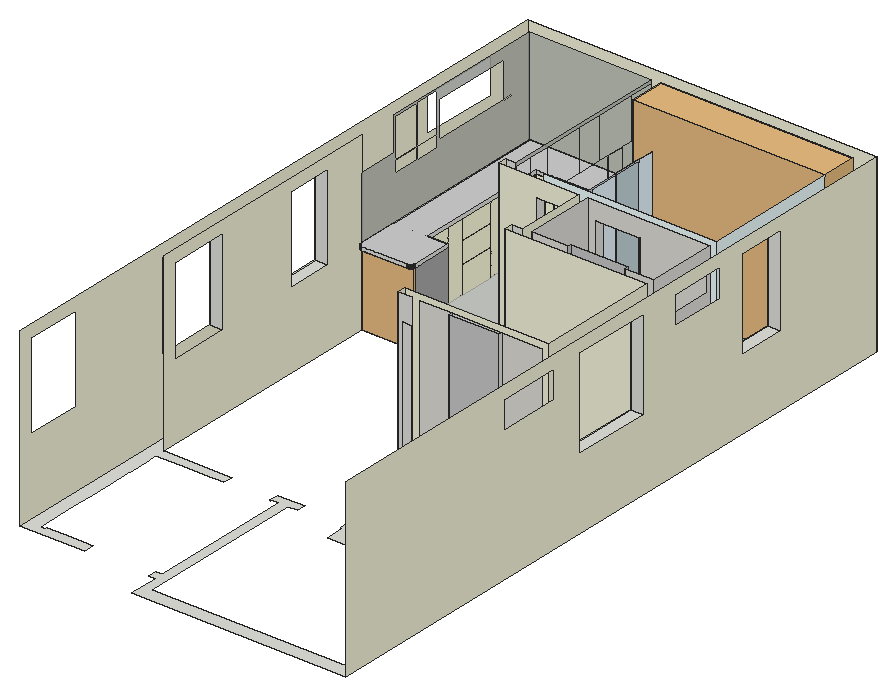
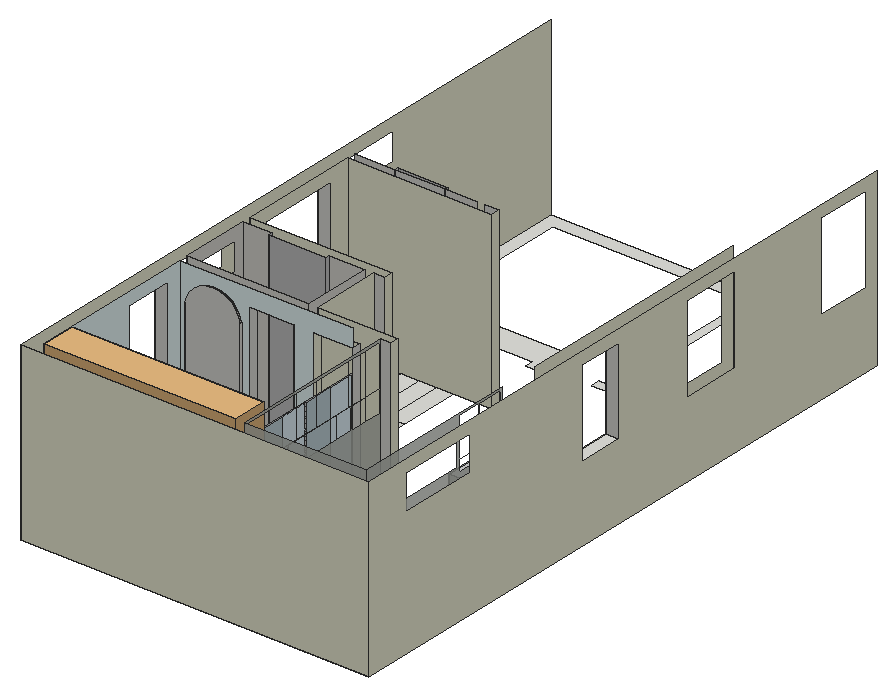
# SketchUp Ruby script. Lengths in inches.
U = 1.inch
M = Sketchup.active_model
def pt(a) = Geom::Point3d.new(a.map { |v| v * U })
def face(e, loops, mat)
  f = e.add_face(loops[0].map { |a| pt(a) })
  loops[1..].each { |l| e.add_face(l.map { |a| pt(a) }).erase! }
  f.material = f.back_material = mat if mat
  f
end
# faces: each face lists its corners as indices into pts; further lists are holes
def faces(e, pts, list, mat = nil) = list.each { |f| face(e, (f[0].is_a?(Array) ? f : [f]).map { |l| l.map { |i| pts[i] } }, mat) }
# xy, xz, yz: faces in a plane at the given z, y or x. An outline is a flat list of corners, or four numbers for a rectangle; further outlines are holes
def ring(l) = l.size == 4 ? [[l[0], l[1]], [l[2], l[1]], [l[2], l[3]], [l[0], l[3]]] : l.each_slice(2).to_a
def flat(e, list, mat, &to3) = list.each { |f| face(e, (f[0].is_a?(Array) ? f : [f]).map { |l| ring(l).map { |u, v| to3.(u, v) } }, mat) }
def xy(e, z, list, mat = nil) = flat(e, list, mat) { |x, y| [x, y, z] }
def xz(e, y, list, mat = nil) = flat(e, list, mat) { |x, z| [x, y, z] }
def yz(e, x, list, mat = nil) = flat(e, list, mat) { |y, z| [x, y, z] }
def lines(e, pts, list) = list.each { |a, b| e.add_line(pt(pts[a]), pt(pts[b])) }
# prism: a flat outline (further loops are holes) pulled along v
def prism(e, loops, v, mat = nil)
  f = face(e, loops, mat); d = Geom::Vector3d.new(v.map { |x| x * U })
  f.pushpull(f.normal.samedirection?(d) ? d.length : -d.length)
end
def box(e, o, s, mat = nil) = prism(e, [[o, [o[0] + s[0], o[1], o[2]], [o[0] + s[0], o[1] + s[1], o[2]], [o[0], o[1] + s[1], o[2]]]], [0, 0, s[2]], mat)
def at(x, y, z, deg = 0) = Geom::Transformation.translation(pt([x, y, z])) * Geom::Transformation.rotation(ORIGIN, Z_AXIS, deg.degrees)
def axes(o, x, y, z) = Geom::Transformation.new([*x, 0, *y, 0, *z, 0, *pt(o).to_a, 1])
def part(name) = M.definitions.add(name)
# library, detail: a bought-in or finely detailed component or shape, given as its bounding box
def library(name, o, s) = part(name).tap { |d| box(d.entities, o, s) }
def detail(e, o, s) = box(e.add_group.entities, o, s)
def put(e, d, t, mat = nil) = e.add_instance(d, t).tap { |i| i.material = mat if mat }
def group(e, t, mat = nil) = e.add_group.tap { |g| g.transformation = t; g.material = mat if mat }.entities
root = M.entities
M.materials.add("[0049_Beige]").color = [245, 245, 220]
M.materials.add("[0054_LightYellow]").color = [255, 255, 224]
M.materials.add("[0092_Azure]").color = [240, 255, 255]
M.materials.add("[0093_AliceBlue]").color = [232, 248, 255]
M.materials.add("[0095_LightBlue]").color = [197, 216, 221]
M.materials.add("[0132_LightGray]").color = [169, 169, 169]
M.materials.add("[Carrera Marble]").color = [207, 207, 207]
M.materials.add("[Formica Laminate Light]").color = [213, 189, 164]
M.materials.add("[Marble Carrara Gold Floor Tile]").color = [225, 223, 217]
M.materials.add("[Ornate Tile 01]").color = [202, 202, 202]
M.materials.add("[Ornate Tile 02]").color = [201, 201, 201]
M.materials.add("[Roofing Slate Tan]").color = [200, 175, 128]
M.materials.add("[Tile Canvas]").color = [188, 192, 184]
M.materials["[Tile Canvas]"].alpha = 0.84
M.materials.add("[Tile Linen]").color = [182, 181, 151]
c1 = library("Slatted panel",[0,0,0],[36.14,50.3,0.5])
c2 = library("Group\#10",[0,-23.9375,0],[132,23.9375,120])
xy(root,0,[[93,0,240,0,240,456,0,456,0,20,44.53,20,44.53,26.8125,41.25,26.8125,41.25,26,41.05,26,41.05,26.8125,29.25,26.8125,29.25,26,29.05,26,29.05,26.8125,12.5625,26.8125,12.5625,26,9.25,26,9.25,45.1875,9,45.1875,9,45.39,9.25,45.39,9.25,55.9,9,55.9,9,56.09,9.5,56.09,9.5,71.78,9,71.78,9,71.98,9.5,71.98,9.5,83.1,9,83.1,9,83.3,9.5,83.3,9.5,102.55,9,102.55,9,102.75,9.5,102.75,9.5,118.43,9,118.43,9,125.5625,30.5625,125.5625,30.5625,126,30.76,126,30.76,125.5625,42.33,125.5625,42.33,126,42.53,126,42.53,125.5625,55.625,125.5625,55.625,132,9,132,9,302.26,45.9375,302.26,45.9375,330,9,330,9,447,93,447,93,426.38,94.59,426.38,95.3125,330,86,330,86,324,112,324,112,447,231,447,231,330,183.21,330,183.21,324,231,324,231,276,211.1875,276,211.1875,278.4375,171.75,278.4375,171.75,276,147,276,147,324,152.79,324,152.79,330,138.73,330,138.73,324,141,324,141,276,133.48,276,133.48,270,231,270,231,186,131.5,186,131.5,180,141,180,141,172.25,147,172.25,147,180,231,180,231,132,147,132,147,137.75,141,137.75,141,132,136,132,136,126,137,126,137,112.75,228.5625,112.75,228.5625,126,231,126,231,9,99,9,99,126,105.75,126,105.75,132,87.5,132,87.5,125.5625,88.16,125.5625,88.16,126,93,126,93,26,88.38,26,88.38,20,93,20],[168.74,177.6875,203.125,180],[157.6875,186,169.6875,228],[169.6875,186,181.6875,228],[181.6875,186,193.6875,228],
  [193.6875,186,205.6875,228],[205.6875,186,231,228],[157.6875,228,169.6875,270],[169.6875,228,181.6875,270],[181.6875,228,193.6875,270],
  [193.6875,228,205.6875,270],[205.6875,228,231,270],[152.79,324,183.21,330],[93,330,93,435,21.45,435,20.73,426.38,94.59,426.38,95.3125,330]])
xy(root,0,[[147,276,171.75,276,171.75,278.4375,211.1875,278.4375,211.1875,276,231,276,231,324,147,324,147,316.89,158.375,316.89,158.375,278.45,147,278.45]],"[Ornate Tile 02]")
xy(root,0,[[93,330,95.3125,330,94.59,426.38,93,426.38]],"[Roofing Slate Tan]")
xy(root,0,[[21.45,330,93,330,93,426.38,20.73,426.38]],"[Tile Canvas]")
xy(root,0,[[112,330,231,447]],"[Tile Linen]")
xy(root,2.8125,[[9,330,9,447,93,447,93,424.375,30.29,424.375,30.29,330]])
xy(root,3.3125,[[30.29,330.5,31.16,348.5],[30.29,349,31.16,361],[30.29,361.5,31.16,385.5],[30.29,386,31.16,401.5625],[30.29,402.0625,31.16,422.875],
  [31.79,423.5625,43.79,424.375],[44.19,423.5625,62.6875,424.375],[63.1875,423.5625,80,424.375],[80.5,423.5625,92.5,424.375]])
xy(root,3.75,[[111.3125,350.49,112,370.8125],[111.3125,392.31,112,411.67],[111.3125,430.5,112,446.4]],"[Carrera Marble]")
xy(root,9.25,[[187.66,330,187.66,346.57,187.71,347.32,187.86,348.06,188.1,348.77,188.43,349.44,188.85,350.07,189.35,350.63,189.91,351.125,190.54,351.54,191.21,351.875,191.92,352.12,192.66,352.26,193.41,352.3125,222.17,352.3125,222.8,352.2,223.42,352.03,224.02,351.78,224.58,351.47,225.1,351.1,225.58,350.67,226.01,350.1875,226.38,349.66,226.69,349.1,226.94,348.51,227.12,347.89,227.23,347.26,227.23,330]],"[Formica Laminate Light]")
xy(root,18.83,[[44.19,423.5625,62.6875,424.375]],"[0054_LightYellow]")
xy(root,19.125,[[44.19,423.5625,62.6875,424.375]])
xy(root,19.39,[[63.1875,423.5625,80,424.375]],"[0054_LightYellow]")
xy(root,19.6875,[[63.1875,423.5625,80,424.375]])
xy(root,21.84,[[30.29,361.5,31.16,385.5],[30.29,402.0625,31.16,422.875]],"[0054_LightYellow]")
xy(root,22.14,[[30.29,361.5,31.16,385.5],[30.29,402.0625,31.16,422.875]])
xy(root,33.89,[[44.19,423.5625,62.6875,424.375]],"[0054_LightYellow]")
xy(root,34.1875,[[44.19,423.5625,62.6875,424.375]])
xy(root,35.64,[[63.1875,423.5625,80,424.375]],"[0054_LightYellow]")
xy(root,35.9375,[[63.1875,423.5625,80,424.375]])
xy(root,36.45,[[30.29,361.5,31.16,385.5]])
xy(root,36.45,[[30.29,402.0625,31.16,422.875]],"[0054_LightYellow]")
xy(root,36.75,[[30.29,361.5,31.16,385.5],[30.29,402.0625,31.16,422.875]])
xy(root,38.6875,[[147,278.45,158.375,316.89]])
xy(root,39.13,[[187.66,330,227.23,330,227.23,347.26,227.12,347.89,226.94,348.51,226.69,349.1,226.38,349.66,226.01,350.1875,225.58,350.67,225.1,351.1,224.58,351.47,224.02,351.78,223.42,352.03,222.8,352.2,222.17,352.3125,193.41,352.3125,192.66,352.26,191.92,352.12,191.21,351.875,190.54,351.54,189.91,351.125,189.35,350.63,188.85,350.07,188.43,349.44,188.1,348.77,187.86,348.06,187.71,347.32,187.66,346.57]],"[Formica Laminate Light]")
xy(root,41.4,[[188.21,330,226,331.8125]])
xy(root,49,[[231,200.3125,240,256],[231,340.4375,240,373.75]])
xy(root,50.625,[[30.29,330.5,31.16,348.5],[30.29,349,31.16,361],[30.29,361.5,31.16,385.5],[30.29,386,31.16,401.5625],[30.29,402.0625,31.16,422.875],
  [31.79,423.5625,43.79,424.375],[44.19,423.5625,62.6875,424.375],[63.1875,423.5625,80,424.375],[80.5,423.5625,92.5,424.375]],"[0054_LightYellow]")
xy(root,51.1,[[11.93,299.125,11.54,299.15,11.17,299.22,10.81,299.35,10.46,299.52,10.14,299.73,9.86,299.98,9.6,300.27,9.39,300.59,9.22,300.93,9.1,301.29,9.03,301.67,9,302.05,9,302.26,45.9375,302.26,45.91,301.85,45.83,301.45,45.7,301.0625,45.52,300.69,45.29,300.35,45.02,300.04,44.71,299.77,44.37,299.55,44,299.36,43.61,299.23,43.21,299.15,42.8,299.125]])
xy(root,51.125,[[9,330,9,447,93,447,93,423.4375,32.05,423.4375,32.05,330]])
xy(root,52.1875,[[0,241.5625,9,273.5]])
xy(root,53.5,[[11.93,299.125,42.8,299.125,43.21,299.15,43.61,299.23,44,299.36,44.37,299.55,44.71,299.77,45.02,300.04,45.29,300.35,45.52,300.69,45.7,301.0625,45.83,301.45,45.91,301.85,45.9375,302.26,45.9375,330,32.05,330,32.05,423.4375,93,423.4375,93,447,9,447,9,302.05,9.03,301.67,9.1,301.29,9.22,300.93,9.39,300.59,9.6,300.27,9.86,299.98,10.14,299.73,10.46,299.52,10.81,299.35,11.17,299.22,11.54,299.15]],"[Carrera Marble]")
xz(root,172.25,[[141,0,147,108]])
xz(root,177.6875,[[168.74,0,203.125,120]],"[Ornate Tile 01]")
xz(root,180,[[131.5,0,141,120],[168.74,0,203.125,120]])
xz(root,180,[[147,0,168.74,120],[203.125,0,231,120]],"[Marble Carrara Gold Floor Tile]")
xz(root,183,[[0,52.1875,9,111.75]])
xz(root,186,[[131.5,0,231,120]],"[0049_Beige]")
xz(root,200.3125,[[231,49,240,111.25]])
xz(root,241.5625,[[0,52.1875,9,111.75]])
xz(root,256,[[231,49,240,111.25]])
xz(root,270,[[133.48,0,231,120]],"[0049_Beige]")
xz(root,273.5,[[0,52.1875,9,111.75]])
xz(root,276,[[133.48,0,141,120]])
xz(root,276,[[147,0,171.75,120],[211.1875,0,231,120]],"[Marble Carrara Gold Floor Tile]")
xz(root,278.4375,[[171.75,0,211.1875,120]],"[Ornate Tile 02]")
xz(root,278.45,[[147,0,158.375,38.6875]])
xz(root,299.125,[[11.93,51.1,42.8,53.5]])
xz(root,302.26,[[9,0,45.9375,51.1]],"[0132_LightGray]")
xz(root,316.89,[[147,0,158.375,38.6875]])
xz(root,324,[[86,0,112,0,112,108,138.73,108,138.73,0,141,0,141,120,86,120]],"[0049_Beige]")
xz(root,324,[[147,0,152.79,0,152.79,108,183.21,108,183.21,0,231,0,231,120,147,120]],"[Marble Carrara Gold Floor Tile]")
xz(root,330,[[9,0,21.45,2.8125],[21.45,0,21.45,2.8125,30.29,2.8125,30.29,51.125,32.05,51.125,32.05,53.5,45.9375,53.5,45.9375,0],[86,0,93,120],[9,2.8125,21.45,51.125],[21.45,2.8125,30.29,51.125]])
xz(root,330,[[[138.73,0,138.73,108,112,108,112,120,231,120,231,0,183.21,0,183.21,108,152.79,108,152.79,0],[188.21,41.4,226,41.4,226,96.52,224.7,100.76,222.46,104.6,219.41,107.8125,215.69,110.24,211.52,111.75,207.11,112.27,202.7,111.75,198.52,110.24,194.81,107.8125,191.75,104.6,189.51,100.76,188.21,96.52],[187.66,9.25,227.23,39.13]]],"[0092_Azure]")
xz(root,330.5,[[30.29,3.3125,31.16,50.625]])
xz(root,331.8125,[[188.21,41.4,188.21,96.52,189.51,100.76,191.75,104.6,194.81,107.8125,198.52,110.24,202.7,111.75,207.11,112.27,211.52,111.75,215.69,110.24,219.41,107.8125,222.46,104.6,224.7,100.76,226,96.52,226,41.4]])
xz(root,340.4375,[[231,49,240,111.25]])
xz(root,348.5,[[30.29,3.3125,31.16,50.625]],"[0054_LightYellow]")
xz(root,349,[[30.29,3.3125,31.16,50.625]])
xz(root,350.49,[[111.3125,3.75,112,92.18]],"[Carrera Marble]")
xz(root,352.3125,[[193.41,9.25,222.17,39.13]],"[Formica Laminate Light]")
xz(root,361,[[30.29,3.3125,31.16,50.625]],"[0054_LightYellow]")
xz(root,361.5,[[30.29,3.3125,31.16,21.84],[30.29,22.14,31.16,36.45],[30.29,36.75,31.16,50.625]])
xz(root,370.8125,[[111.3125,3.75,112,92.18]],"[Carrera Marble]")
xz(root,373.75,[[231,49,240,111.25]])
xz(root,385.5,[[30.29,3.3125,31.16,21.84],[30.29,22.14,31.16,36.45],[30.29,36.75,31.16,50.625]],"[0054_LightYellow]")
xz(root,386,[[30.29,3.3125,31.16,50.625]])
xz(root,392.31,[[111.3125,3.75,112,92.18]])
xz(root,401.5625,[[30.29,3.3125,31.16,50.625]])
xz(root,402.0625,[[30.29,3.3125,31.16,21.84],[30.29,22.14,31.16,36.45],[30.29,36.75,31.16,50.625]])
xz(root,411.67,[[111.3125,3.75,112,92.18]],"[Carrera Marble]")
xz(root,422.875,[[30.29,3.3125,31.16,21.84],[30.29,22.14,31.16,36.45],[30.29,36.75,31.16,50.625]])
xz(root,423.4375,[[32.05,51.125,93,53.5]])
xz(root,423.5625,[[31.79,3.3125,43.79,50.625],[44.19,3.3125,62.6875,18.83],[63.1875,3.3125,80,19.39],[80.5,3.3125,92.5,50.625],[44.19,19.125,62.6875,33.89],
  [63.1875,19.6875,80,35.64],[44.19,34.1875,62.6875,50.625],[63.1875,35.9375,80,50.625]],"[0054_LightYellow]")
xz(root,424.375,[[31.79,3.3125,43.79,50.625],[44.19,3.3125,62.6875,18.83],[63.1875,3.3125,80,19.39],[80.5,3.3125,92.5,50.625],[44.19,19.125,62.6875,33.89],
  [63.1875,19.6875,80,35.64],[44.19,34.1875,62.6875,50.625],[63.1875,35.9375,80,50.625]])
xz(root,430.5,[[111.3125,3.75,112,92.18]])
xz(root,446.4,[[111.3125,3.75,112,92.18]],"[Carrera Marble]")
xz(root,447,[[9,0,93,2.8125],[99,0,112,3.25],[9,2.8125,93,51.125],[99,3.25,112,92.68],[9,51.125,93,53.5]])
xz(root,447,[[9,53.5,93,120]],"[Tile Canvas]")
xz(root,456,[[0,0,240,120]],"[0049_Beige]")
yz(root,0,[[[20,0,456,120],[141.25,52.1875,183,111.75],[29.375,52.1875,67.375,111.75],[241.5625,52.1875,273.5,111.75],[369.625,87.5625,424.25,111.75]]],"[0049_Beige]")
yz(root,9,[[330,0,447,2.8125],[330,2.8125,447,53.5]])
yz(root,9,[[[132,0,302.26,0,302.26,51.1,302.05,51.1,302.05,120,132,120],[141.25,52.1875,183,111.75],[241.5625,52.1875,273.5,111.75]]],"[0049_Beige]")
yz(root,9,[[[302.05,53.5,447,53.5,447,87.5625,367.1875,87.5625,367.1875,83.7,350.25,83.7,350.25,91.26,367.1875,91.26,367.1875,87.5625,369.625,87.5625,369.625,111.75,424.25,111.75,424.25,87.5625,447,87.5625,447,120,330,120,330,96.5,302.05,96.5,302.05,87.5625,331.5,87.5625,331.5,91.26,350.0625,91.26,350.0625,83.7,331.5,83.7,331.5,87.5625,302.05,87.5625],[331.5,91.5625,350.0625,118.3125],[350.25,91.5625,367.1875,118.3125]]],"[Tile Canvas]")
yz(root,30.29,[[330.5,3.3125,348.5,50.625],[349,3.3125,361,50.625],[361.5,3.3125,385.5,21.84],[386,3.3125,401.5625,50.625],[402.0625,3.3125,422.875,21.84],
  [361.5,22.14,385.5,36.45],[402.0625,22.14,422.875,36.45],[361.5,36.75,385.5,50.625],[402.0625,36.75,422.875,50.625]])
yz(root,31.16,[[330.5,3.3125,348.5,50.625],[349,3.3125,361,50.625],[361.5,3.3125,385.5,21.84],[386,3.3125,401.5625,50.625],[402.0625,3.3125,422.875,21.84],
  [361.5,22.14,385.5,36.45],[402.0625,22.14,422.875,36.45],[361.5,36.75,385.5,50.625],[402.0625,36.75,422.875,50.625]],"[0054_LightYellow]")
yz(root,31.79,[[423.5625,3.3125,424.375,50.625]],"[0054_LightYellow]")
yz(root,32.05,[[330,51.125,423.4375,53.5]])
yz(root,43.79,[[423.5625,3.3125,424.375,50.625]],"[0054_LightYellow]")
yz(root,44.19,[[423.5625,34.1875,424.375,50.625]])
yz(root,44.19,[[423.5625,3.3125,424.375,18.83],[423.5625,19.125,424.375,33.89]],"[0054_LightYellow]")
yz(root,45.9375,[[302.26,51.1,330,53.5]])
yz(root,45.9375,[[302.26,0,330,51.1]],"[0132_LightGray]")
yz(root,62.6875,[[423.5625,3.3125,424.375,18.83],[423.5625,19.125,424.375,33.89],[423.5625,34.1875,424.375,50.625]],"[0054_LightYellow]")
yz(root,63.1875,[[423.5625,3.3125,424.375,19.39],[423.5625,19.6875,424.375,35.64],[423.5625,35.9375,424.375,50.625]])
yz(root,80,[[423.5625,3.3125,424.375,19.39],[423.5625,19.6875,424.375,35.64],[423.5625,35.9375,424.375,50.625]],"[0054_LightYellow]")
yz(root,80.5,[[423.5625,3.3125,424.375,50.625]],"[0054_LightYellow]")
yz(root,86,[[324,0,330,120]],"[0049_Beige]")
yz(root,92.5,[[423.5625,3.3125,424.375,50.625]])
yz(root,93,[[[330,0,330,120,447,120,447,53.5,423.4375,53.5,423.4375,51.125,424.375,51.125,424.375,2.8125,435,2.8125,435,0],[402.1,89.4375,429.35,117.625],[357.2,89.4375,384.45,117.625],[367.79,74.375,409.3,89.25],[384.7,89.4375,401.95,117.625],[429.5,89.4375,446.5,117.625],[342.99,89.4375,356.99,117.625],[330.5,89.4375,342.84,117.625],[434.5,74.375,446.5,89.25],[422.1,74.375,434.1,89.25],[409.7,74.375,421.7,89.25],[355.39,74.375,367.39,89.25],[342.99,74.375,354.99,89.25],[330.5,74.375,342.5,89.25]]],"[Tile Canvas]")
yz(root,111.3125,[[350.49,3.75,370.8125,92.18],[392.31,3.75,411.67,92.18],[430.5,3.75,446.4,92.18]],"[0095_LightBlue]")
yz(root,112,[[324,0,330,108]])
yz(root,112,[[330.92,3.75,350.29,92.18],[371.36,3.75,392.11,92.18],[412.17,3.75,430.3,92.18]],"[0093_AliceBlue]")
yz(root,112,[[330,0,447,3.25],[[330,3.25,447,92.68],[371.36,3.75,392.11,92.18],[350.49,3.75,370.8125,92.18],[330.92,3.75,350.29,92.18],[392.31,3.75,411.67,92.18],[412.17,3.75,430.3,92.18],[430.5,3.75,446.4,92.18]]],"[Carrera Marble]")
yz(root,131.5,[[180,0,186,120]],"[0049_Beige]")
yz(root,133.48,[[270,0,276,120]],"[0049_Beige]")
yz(root,138.73,[[324,0,330,108]],"[0049_Beige]")
yz(root,141,[[276,0,324,120]],"[0049_Beige]")
yz(root,147,[[278.45,0,316.89,38.6875]])
yz(root,147,[[276,0,278.45,0,278.45,38.6875,316.89,38.6875,316.89,0,324,0,324,120,276,120]],"[Marble Carrara Gold Floor Tile]")
yz(root,152.79,[[324,0,330,108]])
yz(root,158.375,[[278.45,0,316.89,38.6875]])
yz(root,168.74,[[177.6875,0,180,120]],"[Ornate Tile 01]")
yz(root,171.75,[[276,0,278.4375,120]],"[Ornate Tile 02]")
yz(root,183.21,[[324,0,330,108]])
yz(root,187.66,[[330,9.25,346.57,39.13]],"[Formica Laminate Light]")
yz(root,188.21,[[330,41.4,331.8125,96.52]])
yz(root,203.125,[[177.6875,0,180,120]])
yz(root,211.1875,[[276,0,278.4375,120]],"[Ornate Tile 02]")
yz(root,226,[[330,41.4,331.8125,96.52]])
yz(root,227.23,[[330,9.25,347.26,39.13]],"[Formica Laminate Light]")
yz(root,231,[[[186,0,270,120],[200.3125,49,256,111.25]]],"[0049_Beige]")
yz(root,231,[[[330,0,447,120],[340.4375,49,373.75,111.25]]],"[0092_Azure]")
yz(root,231,[[[276,0,324,120],[282.5625,92,321.125,111.25]]],"[Marble Carrara Gold Floor Tile]")
yz(root,240,[[[0,0,456,120],[200.3125,49,256,111.25],[340.4375,49,373.75,111.25],[135.375,92,178.8125,111.25],[282.5625,92,321.125,111.25]]],"[0049_Beige]")
p = [[187.66,346.57,39.13],[187.71,347.32,39.13],[187.71,347.32,9.25],[187.66,346.57,9.25],[187.86,348.06,39.13],[187.86,348.06,9.25],
  [227.12,347.89,39.13],[227.23,347.26,39.13],[227.23,347.26,9.25],[227.12,347.89,9.25],[226.94,348.51,39.13],[226.94,348.51,9.25],
  [188.1,348.77,39.13],[188.1,348.77,9.25],[226.69,349.1,39.13],[226.69,349.1,9.25],[188.43,349.44,39.13],[188.43,349.44,9.25],
  [226.38,349.66,39.13],[226.38,349.66,9.25],[188.85,350.07,39.13],[188.85,350.07,9.25],[226.01,350.1875,39.13],[226.01,350.1875,9.25],
  [189.35,350.63,39.13],[189.35,350.63,9.25],[225.58,350.67,39.13],[225.58,350.67,9.25],[189.91,351.125,39.13],[189.91,351.125,9.25],
  [225.1,351.1,39.13],[225.1,351.1,9.25],[190.54,351.54,39.13],[190.54,351.54,9.25],[224.58,351.47,39.13],[224.58,351.47,9.25],
  [191.21,351.875,39.13],[191.21,351.875,9.25],[224.02,351.78,39.13],[224.02,351.78,9.25],[223.42,352.03,39.13],[223.42,352.03,9.25],
  [191.92,352.12,39.13],[191.92,352.12,9.25],[222.8,352.2,39.13],[222.8,352.2,9.25],[192.66,352.26,39.13],[192.66,352.26,9.25],
  [222.17,352.3125,39.13],[222.17,352.3125,9.25],[193.41,352.3125,39.13],[193.41,352.3125,9.25],[11.93,299.125,53.5],[11.54,299.15,53.5],
  [11.54,299.15,51.1],[11.93,299.125,51.1],[43.21,299.15,53.5],[42.8,299.125,53.5],[42.8,299.125,51.1],[43.21,299.15,51.1],
  [11.17,299.22,53.5],[10.81,299.35,53.5],[10.81,299.35,51.1],[11.17,299.22,51.1],[43.61,299.23,53.5],[43.61,299.23,51.1],
  [44,299.36,53.5],[44,299.36,51.1],[10.46,299.52,53.5],[10.46,299.52,51.1],[44.37,299.55,53.5],[44.37,299.55,51.1],
  [10.14,299.73,53.5],[10.14,299.73,51.1],[44.71,299.77,53.5],[44.71,299.77,51.1],[9.86,299.98,53.5],[9.86,299.98,51.1],
  [45.02,300.04,53.5],[45.02,300.04,51.1],[9.6,300.27,53.5],[9.6,300.27,51.1],[45.29,300.35,53.5],[45.29,300.35,51.1],
  [9.39,300.59,53.5],[9.39,300.59,51.1],[45.52,300.69,53.5],[45.52,300.69,51.1],[9.22,300.93,53.5],[9.22,300.93,51.1],
  [45.7,301.0625,53.5],[45.7,301.0625,51.1],[9.1,301.29,53.5],[9.1,301.29,51.1],[45.83,301.45,53.5],[45.83,301.45,51.1],
  [9.03,301.67,53.5],[9.03,301.67,51.1],[45.91,301.85,53.5],[45.91,301.85,51.1],[9,302.05,53.5],[9,302.05,51.1],
  [45.9375,302.26,53.5],[45.9375,302.26,51.1],[21.45,330,51.125],[21.45,330,53.5],[30.29,330,51.125],[30.29,330,53.5]]
faces(root,p,[[0,1,2,3],[1,4,5,2],[6,7,8,9],[10,6,9,11],[4,12,13,5],[14,10,11,15],[12,16,17,13],[18,14,15,19],
  [16,20,21,17],[22,18,19,23],[20,24,25,21],[26,22,23,27],[24,28,29,25],[30,26,27,31],[28,32,33,29],[34,30,31,35],
  [32,36,37,33],[38,34,35,39],[40,38,39,41],[36,42,43,37],[44,40,41,45],[42,46,47,43],[48,44,45,49],[46,50,51,47]],"[Formica Laminate Light]")
faces(root,p,[[52,53,54,55],[56,57,58,59],[60,61,62,63],[53,60,63,54],[64,56,59,65],[66,64,65,67],[61,68,69,62],[70,66,67,71],
  [68,72,73,69],[74,70,71,75],[72,76,77,73],[78,74,75,79],[76,80,81,77],[82,78,79,83],[80,84,85,81],[86,82,83,87],
  [84,88,89,85],[90,86,87,91],[88,92,93,89],[94,90,91,95],[92,96,97,93],[98,94,95,99],[96,100,101,97],[102,98,99,103]])
lines(root,p,[[104,105],[106,107]])
g1 = group(root,at(147,276,0))
p = [[0,0,0],[84,0,0],[84,48,0],[36.21,48,0],[5.79,48,0],[0,48,0]]
lines(g1,p,[[0,1],[2,3],[3,4],[4,5],[5,0],[1,2]])
put(root,c1,axes([9.4,302.26,0.4],[1,0,0],[0,0,1],[0,-1,0]))
g2 = group(root,at(9,330,0))
p = [[36.9375,0,0],[0,0,0],[81.6875,0,0],[84,0,0],[84,117,0],[0,117,0]]
lines(g2,p,[[0,1],[2,0],[3,2],[4,3],[5,4],[1,5]])
g3 = group(root,at(9,330,0))
xy(g3,2.8125,[[0,0,12.45,0,12.45,105,84,105,84,117,0,117]])
xz(g3,105,[[12.45,0,84,2.8125]])
yz(g3,12.45,[[0,0,105,2.8125]])
g4 = group(root,at(9,330,2.8125))
xy(g4,48.3125,[[0,0,21.29,0,21.29,94.375,84,94.375,84,117,0,117]])
xz(g4,94.375,[[21.29,0,84,48.3125]],"[0054_LightYellow]")
yz(g4,21.29,[[0,0,94.375,48.3125]])
put(root,c2,at(99,447,0))
